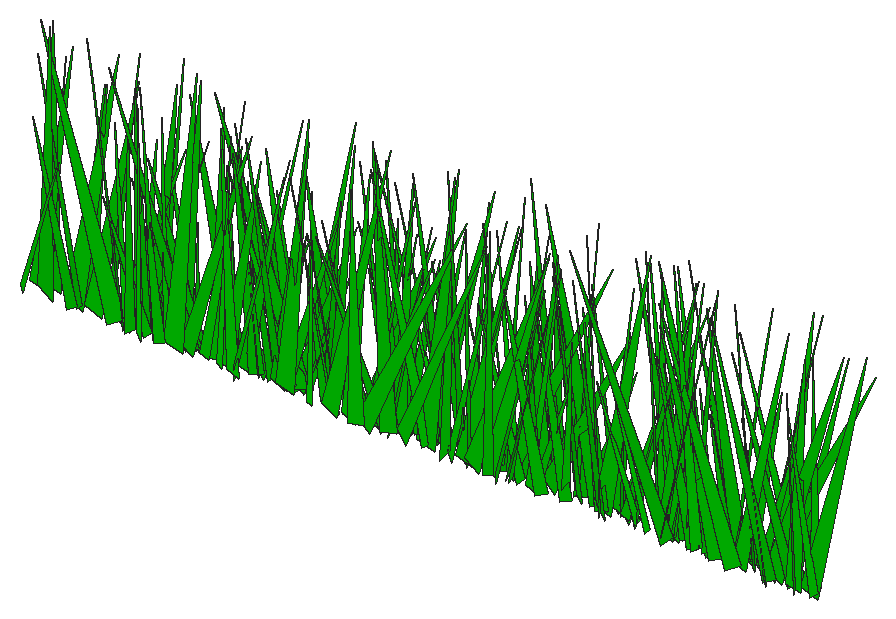
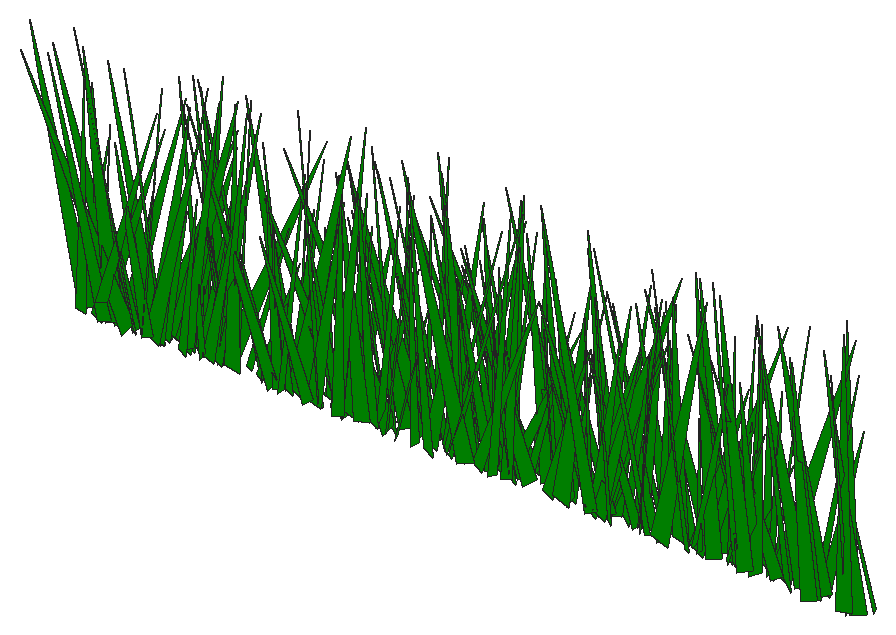
# SketchUp Ruby script. Lengths in inches.
U = 1.inch
M = Sketchup.active_model
def pt(a) = Geom::Point3d.new(a.map { |v| v * U })
def face(e, loops, mat)
  f = e.add_face(loops[0].map { |a| pt(a) })
  loops[1..].each { |l| e.add_face(l.map { |a| pt(a) }).erase! }
  f.material = f.back_material = mat if mat
  f
end
# faces: each face lists its corners as indices into pts; further lists are holes
def faces(e, pts, list, mat = nil) = list.each { |f| face(e, (f[0].is_a?(Array) ? f : [f]).map { |l| l.map { |i| pts[i] } }, mat) }
# xy, xz, yz: faces in a plane at the given z, y or x. An outline is a flat list of corners, or four numbers for a rectangle; further outlines are holes
def ring(l) = l.size == 4 ? [[l[0], l[1]], [l[2], l[1]], [l[2], l[3]], [l[0], l[3]]] : l.each_slice(2).to_a
def flat(e, list, mat, &to3) = list.each { |f| face(e, (f[0].is_a?(Array) ? f : [f]).map { |l| ring(l).map { |u, v| to3.(u, v) } }, mat) }
def xy(e, z, list, mat = nil) = flat(e, list, mat) { |x, y| [x, y, z] }
def xz(e, y, list, mat = nil) = flat(e, list, mat) { |x, z| [x, y, z] }
def yz(e, x, list, mat = nil) = flat(e, list, mat) { |y, z| [x, y, z] }
def lines(e, pts, list) = list.each { |a, b| e.add_line(pt(pts[a]), pt(pts[b])) }
# prism: a flat outline (further loops are holes) pulled along v
def prism(e, loops, v, mat = nil)
  f = face(e, loops, mat); d = Geom::Vector3d.new(v.map { |x| x * U })
  f.pushpull(f.normal.samedirection?(d) ? d.length : -d.length)
end
def box(e, o, s, mat = nil) = prism(e, [[o, [o[0] + s[0], o[1], o[2]], [o[0] + s[0], o[1] + s[1], o[2]], [o[0], o[1] + s[1], o[2]]]], [0, 0, s[2]], mat)
def at(x, y, z, deg = 0) = Geom::Transformation.translation(pt([x, y, z])) * Geom::Transformation.rotation(ORIGIN, Z_AXIS, deg.degrees)
def axes(o, x, y, z) = Geom::Transformation.new([*x, 0, *y, 0, *z, 0, *pt(o).to_a, 1])
def part(name) = M.definitions.add(name)
# library, detail: a bought-in or finely detailed component or shape, given as its bounding box
def library(name, o, s) = part(name).tap { |d| box(d.entities, o, s) }
def detail(e, o, s) = box(e.add_group.entities, o, s)
def put(e, d, t, mat = nil) = e.add_instance(d, t).tap { |i| i.material = mat if mat }
def group(e, t, mat = nil) = e.add_group.tap { |g| g.transformation = t; g.material = mat if mat }.entities
root = M.entities
M.materials.add("[Color G06]").color = [0, 204, 0]
c1 = part("fur_instance\#9")
p = [[0.8125,0,1.79],[0.67,-0.02,1.48],[0,-0.11,0],[0,0.11,0]]
faces(c1.entities,p,[[0,1,2,3]])
put(root,c1,axes([103.76,23.92,4.28],[-4.42176,-0.47384,0.10033],[-3.15087,0.57728,3.00292],[1.27403,-0.21685,7.7749]),"[Color G06]")
put(root,c1,axes([87.62,23.25,4.28],[0.67804,0.71547,0.05759],[5.07732,-0.09434,1.10789],[-0.7399,0.00827,7.65528]),"[Color G06]")
put(root,c1,axes([96.52,23.38,4.28],[3.3844,0.51064,1.9258],[3.53451,-0.50391,1.47424],[-1.60547,-0.03292,7.30528]),"[Color G06]")
put(root,c1,axes([100.07,23.5,4.28],[-1.47417,0.52641,1.3588],[3.79266,0.16613,1.79767],[-0.83244,-0.1753,5.78404]),"[Color G06]")
put(root,c1,axes([87.96,23.49,4.28],[4.85518,-0.52204,0.21187],[-3.35437,-0.59134,4.32478],[1.66845,0.33027,8.07829]),"[Color G06]")
put(root,c1,axes([101.4375,23.8,4.28],[2.62945,-0.37944,0.26273],[-2.61849,-0.36088,-1.33277],[-0.76066,-0.06937,5.49609]),"[Color G06]")
put(root,c1,axes([84.3125,23.48,4.28],[-2.87741,0.18491,1.60193],[1.12828,0.42631,-1.1257],[1.27832,0.03994,4.59942]),"[Color G06]")
put(root,c1,axes([64.55,23.6875,4.28],[3.14372,0.14643,0.49204],[1.09742,-0.40674,-1.75672],[0.08226,-0.16983,4.63175]),"[Color G06]")
put(root,c1,axes([96.36,23.67,4.28],[3.21126,-0.61959,0.94075],[-4.39498,-0.41239,2.31012],[0.90723,0.19533,7.8612]),"[Color G06]")
put(root,c1,axes([90.43,23.68,4.28],[4.64795,0.42794,0.1558],[2.83842,-0.58872,-3.39226],[1.17138,-0.27148,7.60175]),"[Color G06]")
put(root,c1,axes([95.21,23.64,4.28],[3.4759,-0.60332,0.87881],[-4.14978,-0.42387,3.23547],[1.35799,0.24898,7.63763]),"[Color G06]")
put(root,c1,axes([108.5,23.64,4.28],[-4.28972,-0.63093,0.37759],[-4.18755,0.53336,-3.88935],[-1.73207,0.27311,8.46797]),"[Color G06]")
put(root,c1,axes([97.49,23.87,4.28],[4.40916,-0.08799,0.02979],[-0.5859,-0.5776,-2.28566],[-0.2352,-0.21074,6.25226]),"[Color G06]")
put(root,c1,axes([86.02,23.81,4.28],[-3.0997,-0.11922,0.51967],[-0.72125,0.41891,1.42978],[0.57585,-0.11704,4.58809]),"[Color G06]")
put(root,c1,axes([115.39,23.71,4.28],[-2.96655,-0.61597,1.37495],[-4.43582,0.37004,-2.33493],[-0.82589,0.22506,7.60208]),"[Color G06]")
put(root,c1,axes([115.31,23.4375,4.28],[-3.58935,0.03386,0.73191],[-0.01334,0.44803,-2.52721],[0.54644,0.23335,4.74588]),"[Color G06]")
put(root,c1,axes([99.8,23.57,4.28],[-3.13994,-0.26934,2.44575],[-2.4014,0.43197,-1.42191],[0.80122,0.23914,5.32305]),"[Color G06]")
put(root,c1,axes([67.97,23.65,4.28],[-2.03674,-0.43572,1.74389],[-3.28522,0.2291,-1.99485],[-0.57664,0.23377,5.20544]),"[Color G06]")
put(root,c1,axes([97.06,23.38,4.28],[4.88819,0.10169,0.4948],[0.49771,-0.60941,3.40468],[-0.62748,0.30884,6.55518]),"[Color G06]")
put(root,c1,axes([85.55,23.61,4.28],[4.76013,-0.51297,2.32187],[-3.99265,-0.60567,2.91268],[0.06782,0.34741,8.50638]),"[Color G06]")
put(root,c1,axes([113.01,23.59,4.28],[-3.13676,0.64446,0.1265],[4.37802,0.40964,2.75959],[-1.48307,-0.15383,7.87875]),"[Color G06]")
put(root,c1,axes([72.71,23.47,4.28],[-4.5376,0.20348,2.07834],[0.91217,0.63323,-2.67342],[1.79751,0.19233,6.60317]),"[Color G06]")
put(root,c1,axes([99.12,23.64,4.28],[4.48387,-0.20567,1.93916],[-1.74673,-0.62372,1.42281],[-0.89868,0.18615,6.90973]),"[Color G06]")
put(root,c1,axes([94.34,23.92,4.28],[-5.00344,-0.43474,2.33291],[-2.92235,0.73056,1.63902],[1.9016,-0.02116,8.65712]),"[Color G06]")
put(root,c1,axes([65.85,24.06,4.28],[-3.13401,-0.74009,1.24941],[-5.02097,0.45146,2.58731],[1.91224,-0.02753,8.84115]),"[Color G06]")
put(root,c1,axes([101.53,23.74,4.28],[-1.94557,0.43929,1.45349],[3.28728,0.2464,1.27429],[-0.25275,-0.17687,5.38516]),"[Color G06]")
put(root,c1,axes([89.54,23.61,4.28],[1.67635,0.76745,2.44258],[5.5422,-0.27828,1.54748],[-1.49808,-0.17071,8.4582]),"[Color G06]")
put(root,c1,axes([99.52,23.74,4.28],[1.71601,0.29206,0.42477],[2.05227,-0.21803,-1.29917],[0.5055,-0.10628,3.83254]),"[Color G06]")
put(root,c1,axes([89.2,23.71,4.28],[-3.17243,-0.3846,0.3379],[-2.4927,0.37632,-3.07247],[-1.20191,0.23469,5.48027]),"[Color G06]")
put(root,c1,axes([79.1,23.47,4.28],[-3.88047,0.5135,0.37686],[3.53843,0.53204,-1.89308],[1.05057,0.10475,7.76809]),"[Color G06]")
put(root,c1,axes([106.99,23.83,4.28],[-3.27739,0.15455,0.50212],[1.15767,0.4411,1.28251],[0.03212,-0.12843,5.00922]),"[Color G06]")
put(root,c1,axes([92.07,23.81,4.28],[-4.76782,0.40055,1.23249],[2.9884,0.64053,1.9098],[0.02087,-0.21205,8.09697]),"[Color G06]")
put(root,c1,axes([110.25,23.94,4.28],[-4.93266,0.3144,3.52064],[2.88848,0.69769,1.88271],[1.5129,-0.307,7.88415]),"[Color G06]")
put(root,c1,axes([86.92,23.54,4.28],[-3.11873,0.60481,1.68165],[4.02012,0.46211,-2.43793],[1.97892,0.0144,7.60284]),"[Color G06]")
put(root,c1,axes([91.9375,23.82,4.28],[2.23973,0.72867,3.31468],[5.67106,-0.27248,-1.67866],[0.25161,-0.34488,8.32953]),"[Color G06]")
put(root,c1,axes([77.99,23.7,4.28],[4.45987,-0.08103,2.80629],[-1.00044,-0.65243,1.38749],[-1.69185,0.17221,6.57718]),"[Color G06]")
put(root,c1,axes([98.33,23.93,4.28],[-2.97416,0.28695,1.48091],[2.27672,0.35452,2.32259],[-0.18099,-0.25576,4.8809]),"[Color G06]")
put(root,c1,axes([117.11,23.66,4.28],[-3.9042,-0.02748,2.25127],[-0.71556,0.54423,-2.00895],[1.34005,0.21056,5.4863]),"[Color G06]")
put(root,c1,axes([87.95,23.87,4.28],[-3.50346,-0.29959,0.4492],[-2.16405,0.47706,-1.1511],[-0.15203,0.11332,6.03351]),"[Color G06]")
put(root,c1,axes([73.9375,23.68,4.28],[-0.02746,0.46538,0.10392],[3.2614,0.00167,1.06404],[-0.7115,-0.01029,4.87332]),"[Color G06]")
put(root,c1,axes([89.79,23.79,4.28],[-0.35765,0.44554,1.32908],[3.2079,0.01481,1.35783],[-0.84188,-0.13283,4.60927]),"[Color G06]")
put(root,c1,axes([118.22,23.98,4.28],[-3.19332,0.2203,1.89852],[1.9457,0.42584,1.63399],[0.56895,-0.21983,5.06788]),"[Color G06]")
put(root,c1,axes([117.85,24.04,4.28],[3.21385,-0.68495,0.78254],[-4.86617,-0.42401,2.0078],[0.84955,0.16245,8.54019]),"[Color G06]")
put(root,c1,axes([111.23,24.18,4.28],[1.26514,-0.68431,1.08413],[-4.3561,-0.20319,-3.37851],[-2.37333,0.00817,6.77897]),"[Color G06]")
put(root,c1,axes([109.63,24.04,4.28],[3.23534,-0.22781,1.37763],[-1.49286,-0.46788,-1.05646],[-1.13576,-0.03396,5.31294]),"[Color G06]")
put(root,c1,axes([71.97,23.6,4.28],[2.65898,0.50873,0.39153],[3.30744,-0.3537,2.62108],[-1.56181,0.11708,6.21722]),"[Color G06]")
put(root,c1,axes([78.24,23.88,4.28],[0.46601,0.60716,2.44774],[4.51254,-0.00324,-1.82685],[1.13024,-0.23742,6.28455]),"[Color G06]")
put(root,c1,axes([81.71,24.15,4.28],[-4.21965,-0.44122,0.67658],[-3.07984,0.58922,1.23426],[0.85497,-0.05507,7.78541]),"[Color G06]")
put(root,c1,axes([73.33,24.17,4.28],[-4.90448,0.08045,3.27223],[1.34534,0.68942,2.55703],[1.82111,-0.29264,6.92354]),"[Color G06]")
put(root,c1,axes([89.38,24.25,4.28],[1.1707,-0.82951,0.612],[-5.88988,-0.16994,-1.29294],[-0.929,0.03211,8.96846]),"[Color G06]")
put(root,c1,axes([113.16,23.97,4.28],[4.07167,-0.49988,1.52813],[-3.72743,-0.54327,1.76992],[0.04742,0.21807,7.9123]),"[Color G06]")
put(root,c1,axes([94.97,23.6875,4.28],[4.14644,0.35157,2.25261],[1.9006,-0.59833,2.91269],[-2.23961,0.14314,6.64228]),"[Color G06]")
put(root,c1,axes([87.83,24.11,4.28],[5.1232,0.20366,1.42002],[1.69092,-0.6804,-2.41716],[-0.42021,-0.25491,7.58629]),"[Color G06]")
put(root,c1,axes([94.58,23.74,4.28],[2.45833,0.71801,0.27765],[5.09389,-0.33438,-1.41188],[0.77401,-0.07984,8.40999]),"[Color G06]")
put(root,c1,axes([93.68,23.68,4.28],[5.80096,-0.01851,1.26512],[-0.45997,-0.74883,3.45243],[-0.7229,0.32792,7.95539]),"[Color G06]")
put(root,c1,axes([108.4,24.14,4.28],[5.37383,-0.30532,1.30049],[-2.09826,-0.75762,-1.06512],[-1.07163,-0.04762,8.607]),"[Color G06]")
put(root,c1,axes([85.29,24.11,4.28],[-4.68156,-0.04223,0.93887],[-0.16996,0.6457,1.44358],[0.67636,-0.13007,6.86134]),"[Color G06]")
put(root,c1,axes([89.65,23.63,4.28],[4.83158,0.28922,0.16745],[1.85445,-0.61846,3.18786],[-0.93568,0.26774,7.18276]),"[Color G06]")
put(root,c1,axes([88.24,23.99,4.28],[3.31274,-0.40924,0.39635],[-2.82575,-0.4254,2.29897],[0.83572,0.18383,6.20224]),"[Color G06]")
put(root,c1,axes([72.9375,23.91,4.28],[-1.24194,0.38027,0.07727],[2.44966,0.15203,2.00087],[-1.19937,-0.08325,4.00668]),"[Color G06]")
put(root,c1,axes([79.1,23.5625,4.28],[5.74462,0.11844,0.75404],[0.44151,-0.67914,4.74091],[-0.88377,0.4306,7.26984]),"[Color G06]")
put(root,c1,axes([80.09,24.22,4.28],[0.95988,-0.65182,0.91207],[-4.57913,-0.14955,-1.51282],[-1.11956,0.05284,6.96963]),"[Color G06]")
put(root,c1,axes([94.25,24.21,4.28],[5.80567,-0.15792,0.06654],[-1.1003,-0.79313,-1.78664],[-0.27167,-0.16245,8.65812]),"[Color G06]")
put(root,c1,axes([75.82,24.12,4.28],[-3.95512,-0.62765,0.07684],[-4.31073,0.52539,-2.64285],[-1.29596,0.16792,8.55639]),"[Color G06]")
put(root,c1,axes([75.58,23.93,4.28],[3.478,0.57392,0.58913],[4.0545,-0.45937,-2.06023],[0.80974,-0.16499,7.78551]),"[Color G06]")
put(root,c1,axes([110.01,23.95,4.28],[-0.95496,0.51654,1.25604],[3.66451,0.09348,1.80706],[-0.99968,-0.15076,5.42424]),"[Color G06]")
put(root,c1,axes([103.78,23.77,4.28],[-5.53145,-0.03072,3.00833],[-0.94951,0.76053,-3.00777],[1.78842,0.30877,7.70763]),"[Color G06]")
put(root,c1,axes([97.8,23.74,4.28],[5.24647,0.3102,0.91221],[1.95299,-0.70985,2.63934],[-1.22757,0.19642,8.0977]),"[Color G06]")
put(root,c1,axes([81.65,24.09,4.28],[-1.68321,-0.63032,3.60073],[-4.72987,0.32699,1.63664],[1.96588,0.24705,7.02071]),"[Color G06]")
put(root,c1,axes([85.28,24.21,4.28],[4.35517,0.42056,3.49805],[3.68826,-0.59132,-2.09053],[-0.98529,-0.35452,7.63655]),"[Color G06]")
put(root,c1,axes([73.95,24.23,4.28],[-4.20785,0.08472,3.23099],[1.23213,0.6224,1.70972],[1.87733,-0.21861,6.11981]),"[Color G06]")
put(root,c1,axes([68.25,23.98,4.28],[-4.75983,-0.23493,1.48367],[-1.89001,0.64617,-1.79059],[0.50169,0.20537,7.33088]),"[Color G06]")
put(root,c1,axes([82.25,23.94,4.28],[0.14072,0.78556,2.23618],[5.78272,0.00736,-1.10992],[0.73109,-0.20943,8.34876]),"[Color G06]")
put(root,c1,axes([70.74,23.96,4.28],[-2.81685,0.77509,1.03789],[5.34422,0.33938,3.28429],[-1.67853,-0.2202,8.71499]),"[Color G06]")
put(root,c1,axes([105.72,24.26,4.28],[6.03573,0.19538,0.91676],[1.52571,-0.79357,-3.00977],[-0.10748,-0.29317,8.75796]),"[Color G06]")
put(root,c1,axes([76.7,24.04,4.28],[4.14069,-0.3042,1.59392],[-2.38059,-0.56649,1.39463],[-0.47851,0.186,6.85445]),"[Color G06]")
put(root,c1,axes([93.43,23.59,4.28],[4.51513,0.60583,0.41259],[3.7387,-0.56804,4.42505],[-2.23019,0.27427,8.25348]),"[Color G06]")
put(root,c1,axes([74.82,23.76,4.28],[-1.38709,0.84486,0.43069],[5.94579,0.19754,-1.74016],[1.19934,-0.0022,9.12501]),"[Color G06]")
put(root,c1,axes([115.25,24.26,4.28],[2.7128,-0.72957,0.38909],[-4.98924,-0.34739,2.87559],[1.59646,0.15408,8.32558]),"[Color G06]")
put(root,c1,axes([116.68,24.08,4.28],[-3.2046,-0.4911,1.19305],[-3.50191,0.3863,-2.74461],[-0.88153,0.25071,6.56599]),"[Color G06]")
put(root,c1,axes([116.86,23.92,4.28],[-1.96966,0.61703,1.4597],[4.38052,0.29727,-1.23192],[1.15956,-0.07492,7.13333]),"[Color G06]")
put(root,c1,axes([72.83,24.04,4.28],[-3.97739,-0.29762,2.82201],[-2.5434,0.57464,-1.04552],[1.28512,0.21616,6.66477]),"[Color G06]")
put(root,c1,axes([79.35,24.1875,4.28],[3.00418,-0.47702,0.93058],[-3.47321,-0.40631,1.12042],[0.16327,0.13397,6.71149]),"[Color G06]")
put(root,c1,axes([111.8,23.89,4.28],[-1.29344,0.84878,0.79293],[5.80688,0.14725,3.05159],[-1.90026,-0.12775,8.78543]),"[Color G06]")
put(root,c1,axes([71.31,23.87,4.28],[-5.90892,-0.02345,1.82867],[-0.59143,0.78582,-3.11133],[1.08422,0.30087,8.26891]),"[Color G06]")
put(root,c1,axes([107.98,24.17,4.28],[-1.6969,-0.66107,3.66484],[-4.96681,0.32694,1.63749],[1.95391,0.25695,7.34524]),"[Color G06]")
put(root,c1,axes([101.95,24.34,4.28],[-4.53463,-0.29903,1.2541],[-1.9433,0.63558,1.71338],[1.23538,-0.09783,7.29853]),"[Color G06]")
put(root,c1,axes([91.7,24.14,4.28],[4.00061,0.37651,1.4035],[2.84316,-0.54751,-1.22995],[-0.29796,-0.16909,7.10797]),"[Color G06]")
put(root,c1,axes([103.66,24.17,4.28],[3.38788,-0.65218,2.06153],[-4.86451,-0.43592,2.01534],[0.33594,0.26487,8.39269]),"[Color G06]")
put(root,c1,axes([105.99,24.22,4.28],[-2.78166,0.15925,0.37421],[1.15011,0.35652,1.66772],[-0.21018,-0.15675,4.17325]),"[Color G06]")
put(root,c1,axes([72.01,24.55,4.28],[-3.33455,-0.67078,0.05543],[-4.52992,0.43997,2.90772],[1.61888,-0.15055,8.2505]),"[Color G06]")
put(root,c1,axes([94.26,24.36,4.28],[-0.13404,-0.5905,0.32918],[-4.10367,0.01033,-1.60494],[-1.06801,0.03444,6.1254]),"[Color G06]")
put(root,c1,axes([93.22,24.11,4.28],[2.69734,0.56692,4.08087],[4.14738,-0.4956,1.78571],[-2.60448,-0.20206,7.06994]),"[Color G06]")
put(root,c1,axes([112.48,24.1,4.28],[0.44033,0.38785,1.46671],[2.7488,-0.10412,1.31954],[-1.06918,-0.10796,3.99652]),"[Color G06]")
put(root,c1,axes([107.65,23.99,4.28],[-5.5403,0.05647,2.73888],[-0.01512,0.79511,-1.95164],[1.8767,0.17312,8.06984]),"[Color G06]")
put(root,c1,axes([110.02,24.1875,4.28],[-2.80623,-0.32436,1.03163],[-2.42548,0.37883,-1.05515],[0.06282,0.1374,5.34443]),"[Color G06]")
put(root,c1,axes([110.86,24.04,4.28],[1.67743,0.4586,1.57953],[3.091,-0.27241,1.75306],[-1.54216,-0.04718,5.23177]),"[Color G06]")
put(root,c1,axes([71.51,23.89,4.28],[-4.04072,0.31011,0.4785],[1.94439,0.52868,-2.68227],[1.12578,0.19995,6.35012]),"[Color G06]")
put(root,c1,axes([76.14,24.43,4.28],[-0.24287,-0.60224,0.05194],[-3.97966,0.02932,-2.51445],[-1.67799,0.01763,5.95597]),"[Color G06]")
put(root,c1,axes([82.48,24.21,4.28],[-3.70641,0.36206,0.20705],[2.50946,0.48932,2.05325],[-0.68047,-0.16754,6.44427]),"[Color G06]")
put(root,c1,axes([89.98,23.95,4.28],[2.53746,0.67643,0.76922],[4.8021,-0.3606,1.04271],[-0.85753,-0.01778,8.11522]),"[Color G06]")
put(root,c1,axes([107.79,24.01,4.28],[5.57284,0.13794,0.65542],[0.872,-0.76247,1.87212],[-0.64065,0.16208,8.24945]),"[Color G06]")
put(root,c1,axes([87.6,24.25,4.28],[0.47795,-0.63035,2.81125],[-4.26138,0.07622,3.58146],[2.41093,0.25967,5.77301]),"[Color G06]")
put(root,c1,axes([109.71,24.4375,4.28],[5.26442,0.2026,3.00847],[2.10047,-0.71429,-2.68441],[-1.32319,-0.32783,7.70816]),"[Color G06]")
put(root,c1,axes([86.18,24.02,4.28],[3.35523,0.15927,1.48894],[0.67364,-0.45902,2.24947],[-1.35764,0.16585,4.79587]),"[Color G06]")
put(root,c1,axes([84.6,24.56,4.28],[-3.53955,-0.4625,1.77798],[-2.55504,0.4988,3.54342],[2.42647,-0.14944,6.32475]),"[Color G06]")
put(root,c1,axes([108.4,24.06,4.28],[2.85302,0.22323,0.31304],[1.4961,-0.38784,1.31363],[-0.60692,0.09334,4.70968]),"[Color G06]")
put(root,c1,axes([99.51,24.53,4.28],[1.83226,-0.64786,0.63338],[-4.51586,-0.26223,-1.63219],[-1.17129,-0.00243,7.28364]),"[Color G06]")
put(root,c1,axes([107.62,24.47,4.28],[3.40961,-0.59768,1.76257],[-4.19822,-0.50108,-1.37797],[-1.46176,0.04499,8.06882]),"[Color G06]")
put(root,c1,axes([70.86,24.14,4.28],[2.22558,0.57585,0.10584],[3.884,-0.28799,-2.43788],[1.40456,-0.11607,6.5737]),"[Color G06]")
put(root,c1,axes([105.06,24.36,4.28],[1.13649,-0.34888,0.14792],[-2.38613,-0.14632,1.30843],[0.75879,0.06243,3.89301]),"[Color G06]")
put(root,c1,axes([103.67,24.1,4.28],[-0.25908,0.58691,0.69136],[4.16504,0.02369,1.17641],[-0.76243,-0.07004,6.19165]),"[Color G06]")
put(root,c1,axes([82.12,24.18,4.28],[2.44072,0.50646,0.29773],[3.53476,-0.32235,-1.73642],[0.85818,-0.11269,6.30536]),"[Color G06]")
put(root,c1,axes([108.93,24.33,4.28],[2.24868,0.56717,4.90446],[4.45908,-0.46803,1.65075],[-2.72551,-0.29777,6.74715]),"[Color G06]")
put(root,c1,axes([89.91,24.27,4.28],[-1.46855,0.37647,2.59508],[2.81091,0.27939,-1.10285],[1.54993,-0.15,4.45894]),"[Color G06]")
put(root,c1,axes([80.26,24.17,4.28],[-4.25896,0.0037,1.67876],[-0.22869,0.59833,-1.44754],[1.10003,0.13872,6.19867]),"[Color G06]")
put(root,c1,axes([72.65,24.21,4.28],[4.88637,-0.04573,0.00223],[-0.32317,-0.67087,1.2806],[0.05591,0.11923,7.20658]),"[Color G06]")
put(root,c1,axes([89.29,24.38,4.28],[-5.24248,0.04478,1.83981],[0.49837,0.74201,1.09733],[1.17051,-0.11535,7.77289]),"[Color G06]")
put(root,c1,axes([75.875,24.48,4.28],[-2.24038,-0.26321,0.86732],[-1.57877,0.31225,1.77614],[1.18622,-0.08154,4.00198]),"[Color G06]")
put(root,c1,axes([74.85,24.51,4.28],[-1.91116,-0.75759,2.04927],[-5.3213,0.30867,2.02337],[1.75504,0.11091,8.36642]),"[Color G06]")
put(root,c1,axes([69.14,24.09,4.28],[0.579,0.75453,0.83722],[5.29026,-0.0598,-1.98086],[1.267,-0.0951,7.88832]),"[Color G06]")
put(root,c1,axes([114.26,24.38,4.28],[2.59253,0.30827,1.20995],[2.32375,-0.30812,-2.10387],[0.37782,-0.22023,4.63724]),"[Color G06]")
put(root,c1,axes([82.96,24.39,4.28],[-1.38086,0.76135,3.96462],[5.49209,-0.00487,4.38025],[-2.58531,-0.41699,7.18758]),"[Color G06]")
put(root,c1,axes([91.64,24.43,4.28],[1.0598,-0.77126,2.26061],[-5.70279,-0.11944,1.29104],[0.59717,0.22817,8.31709]),"[Color G06]")
put(root,c1,axes([80.19,24.41,4.28],[2.60531,0.35339,1.14941],[2.53595,-0.28952,-2.61435],[0.76346,-0.24426,4.76163]),"[Color G06]")
put(root,c1,axes([81.96,24.5,4.28],[3.41419,-0.08749,0.82931],[-0.44869,-0.46527,-1.51243],[-0.70726,-0.12717,4.96286]),"[Color G06]")
put(root,c1,axes([97.05,24.6,4.28],[-5.02139,-0.21694,1.58454],[-1.20028,0.69334,2.40803],[1.45038,-0.17728,7.47865]),"[Color G06]")
put(root,c1,axes([91.88,24.33,4.28],[2.77879,-0.37485,1.18531],[-2.78928,-0.35463,1.72315],[0.27425,0.19135,5.51551]),"[Color G06]")
put(root,c1,axes([103.68,24.56,4.28],[4.87694,-0.23802,1.00121],[-1.53442,-0.67507,-1.74024],[-1.00389,-0.12447,7.52385]),"[Color G06]")
put(root,c1,axes([72.67,24.62,4.28],[-1.68628,-0.76405,1.51596],[-5.21632,0.26842,2.57965],[1.95979,0.05702,8.17059]),"[Color G06]")
put(root,c1,axes([112.87,24.48,4.28],[-0.20959,-0.70204,1.9888],[-5.08615,-0.01224,-1.6936],[-1.11707,0.18745,7.33803]),"[Color G06]")
put(root,c1,axes([90.09,24.22,4.28],[-3.08228,0.10643,1.63971],[0.41569,0.44184,-1.54903],[1.27019,0.11367,4.48591]),"[Color G06]")
put(root,c1,axes([89.3,24.1875,4.28],[2.52607,0.50631,1.15314],[3.55794,-0.36736,1.11909],[-1.0582,-0.02651,6.51534]),"[Color G06]")
put(root,c1,axes([84.72,24.3,4.28],[-0.12173,0.39354,1.06739],[2.8061,-0.01067,1.16687],[-0.77498,-0.10046,4.05743]),"[Color G06]")
put(root,c1,axes([81.08,24.23,4.28],[-4.56452,-0.29537,2.19069],[-2.51467,0.6011,-2.39369],[0.55824,0.29257,7.12968]),"[Color G06]")
put(root,c1,axes([113.93,24.22,4.28],[-5.20587,0.01683,2.28709],[-0.21277,0.7393,-1.70684],[1.5202,0.16111,7.59318]),"[Color G06]")
put(root,c1,axes([78.3125,24.59,4.28],[1.77061,-0.3364,0.00566],[-2.29751,-0.23534,-1.35994],[-0.73568,-0.07467,4.26068]),"[Color G06]")
put(root,c1,axes([96.88,24.25,4.28],[5.28378,0.28872,2.31783],[1.94356,-0.76763,1.0874],[-1.7072,0.01968,8.41165]),"[Color G06]")
put(root,c1,axes([93.25,24.34,4.28],[-5.27753,-0.16651,0.64258],[-1.25211,0.72497,-1.39083],[0.20709,0.14,7.96653]),"[Color G06]")
put(root,c1,axes([104.87,24.54,4.28],[4.77572,0.49743,1.11177],[3.43362,-0.55705,-4.31574],[1.22007,-0.37941,7.79392]),"[Color G06]")
put(root,c1,axes([97.07,24.32,4.28],[4.79289,-0.54612,0.26122],[-3.49017,-0.5769,4.49452],[1.78527,0.33833,8.0854]),"[Color G06]")
put(root,c1,axes([74.07,24.36,4.28],[-3.17448,-0.11322,0.23901],[-0.82688,0.43055,-1.10362],[-0.03224,0.10526,4.77124]),"[Color G06]")
put(root,c1,axes([82.69,24.47,4.28],[2.33123,-0.51415,0.6025],[-3.48876,-0.28142,2.56592],[1.25924,0.17216,5.99355]),"[Color G06]")
put(root,c1,axes([83.52,24.34,4.28],[3.1756,-0.08624,0.01822],[-0.5964,-0.4245,1.37321],[0.16417,0.12607,4.63625]),"[Color G06]")
put(root,c1,axes([67.75,24.15,4.28],[-1.38649,0.78643,1.37925],[5.32474,0.22586,-2.83744],[2.07494,-0.0541,8.2031]),"[Color G06]")
put(root,c1,axes([88.42,24.64,4.28],[4.36526,-0.23296,0.20805],[-1.59442,-0.59367,-1.63613],[-0.51784,-0.13589,6.79137]),"[Color G06]")
put(root,c1,axes([76.13,24.4,4.28],[-2.66554,0.37875,1.08816],[2.81202,0.35849,1.05252],[-0.01059,-0.14124,5.58952]),"[Color G06]")
put(root,c1,axes([108.48,24.2,4.28],[-5.16678,0.37264,1.09738],[2.48992,0.7193,-1.87161],[1.21674,0.1104,8.48997]),"[Color G06]")
put(root,c1,axes([117.87,24.57,4.28],[3.74107,-0.37673,2.34111],[-2.61505,-0.56423,-1.09559],[-1.70699,0.03874,6.80924]),"[Color G06]")
put(root,c1,axes([99.76,24.48,4.28],[2.59035,-0.55824,0.42092],[-3.4618,-0.28717,3.83693],[2.03021,0.2226,6.00545]),"[Color G06]")
put(root,c1,axes([88.82,24.7,4.28],[-3.22812,-0.54475,0.98114],[-3.78111,0.45894,1.48288],[1.1813,-0.01967,7.42754]),"[Color G06]")
put(root,c1,axes([85.08,24.77,4.28],[1.20094,-0.69998,0.22186],[-4.81923,-0.16662,-2.11853],[-1.41236,-0.02665,7.41747]),"[Color G06]")
put(root,c1,axes([77.41,24.15,4.28],[1.8711,0.73779,0.25526],[5.22971,-0.26154,1.21065],[-0.82038,0.01546,8.29974]),"[Color G06]")
put(root,c1,axes([109.28,24.46,4.28],[-0.64188,-0.41869,1.99706],[-3.19851,0.03596,-1.43024],[-0.75516,0.20356,4.36034]),"[Color G06]")
put(root,c1,axes([113.04,24.59,4.28],[-1.45611,-0.63623,1.18033],[-4.50671,0.16822,-2.00258],[-1.06319,0.1583,6.87212]),"[Color G06]")
put(root,c1,axes([101.55,24.62,4.28],[5.68597,-0.15459,2.28079],[-0.94383,-0.81834,-1.11573],[-1.63309,-0.06528,8.58592]),"[Color G06]")
put(root,c1,axes([103.21,24.45,4.28],[-0.30341,-0.74822,4.31308],[-5.78645,-0.09071,-2.71692],[-1.90674,0.39434,7.55878]),"[Color G06]")
put(root,c1,axes([114.16,24.62,4.28],[6.21125,0.03539,0.68397],[0.32411,-0.85696,-1.48061],[-0.41086,-0.14097,9.17218]),"[Color G06]")
put(root,c1,axes([92.7,24.63,4.28],[-6.11596,0.00801,0.18506],[0.07684,0.84166,1.485],[0.11283,-0.13873,9.01972]),"[Color G06]")
put(root,c1,axes([72.22,24.26,4.28],[-1.51163,0.56845,0.29749],[3.94501,0.21109,-1.55883],[1.04613,0.02536,6.30828]),"[Color G06]")
put(root,c1,axes([104.84,24.38,4.28],[3.02767,0.17863,1.75593],[0.99933,-0.44812,1.38786],[-1.42219,0.0654,4.71336]),"[Color G06]")
put(root,c1,axes([104.41,24.61,4.28],[-1.56448,-0.47238,1.89664],[-3.40137,0.25773,1.10655],[1.23146,0.11174,5.4659]),"[Color G06]")
put(root,c1,axes([78.18,24.8,4.28],[-2.99438,-0.47283,0.61069],[-3.15503,0.41198,2.0859],[1.30766,-0.08872,6.43114]),"[Color G06]")
put(root,c1,axes([98.7,24.64,4.28],[1.02071,-0.66769,1.64388],[-4.88613,-0.12165,1.10111],[0.51181,0.17025,7.23372]),"[Color G06]")
put(root,c1,axes([114.65,24.59,4.28],[4.30111,0.62233,0.51364],[3.90217,-0.48876,-4.96217],[2.19291,-0.35091,7.82249]),"[Color G06]")
put(root,c1,axes([65.83,24.72,4.28],[-2.22261,-0.73075,1.85559],[-5.24794,0.33594,1.15639],[1.20933,0.11479,8.42855]),"[Color G06]")
put(root,c1,axes([65.07,24.47,4.28],[-0.27247,0.69648,2.85566],[5.16293,0.10377,-1.80691],[1.39325,-0.24832,7.25428]),"[Color G06]")
put(root,c1,axes([86.08,24.64,4.28],[-1.38281,-0.46241,0.5709],[-3.21868,0.16943,-1.64961],[-0.88454,0.10636,5.11011]),"[Color G06]")
put(root,c1,axes([104.08,24.8125,4.28],[-4.21332,-0.36521,0.87336],[-2.38452,0.57913,2.12352],[1.23077,-0.12821,7.10395]),"[Color G06]")
put(root,c1,axes([100.29,24.53,4.28],[1.34174,0.44683,1.48181],[3.30261,-0.14997,-1.48482],[0.58603,-0.17784,4.97514]),"[Color G06]")
put(root,c1,axes([97.71,24.35,4.28],[-4.63969,0.27239,1.20043],[1.76392,0.64842,-1.67346],[1.16169,0.10335,7.33542]),"[Color G06]")
put(root,c1,axes([82.87,24.33,4.28],[-1.5666,0.6708,0.25359],[4.75874,0.2121,1.21843],[-0.72375,-0.05742,7.46243]),"[Color G06]")
put(root,c1,axes([110.88,24.27,4.28],[-4.99429,0.47167,0.3424],[3.29433,0.68861,-1.63585],[0.80075,0.10885,8.86552]),"[Color G06]")
put(root,c1,axes([89.67,24.84,4.28],[-4.39266,-0.51899,1.29354],[-3.50033,0.62028,2.037],[1.53252,-0.07083,8.36023]),"[Color G06]")
put(root,c1,axes([91.59,24.74,4.28],[3.81314,-0.69495,0.29072],[-4.91499,-0.5178,1.81179],[0.84725,0.12391,9.20196]),"[Color G06]")
put(root,c1,axes([112.41,24.38,4.28],[5.39636,0.2395,1.29928],[1.55361,-0.7549,1.57161],[-1.13663,0.10524,8.31671]),"[Color G06]")
put(root,c1,axes([90.05,24.48,4.28],[1.46374,0.50485,0.97675],[3.6356,-0.18349,-1.27539],[0.5631,-0.12767,5.69547]),"[Color G06]")
put(root,c1,axes([101.93,24.68,4.28],[-1.36562,-0.58579,1.44092],[-4.28918,0.17083,-1.10233],[-0.42407,0.1586,6.50926]),"[Color G06]")
put(root,c1,axes([92.11,24.29,4.28],[3.38951,0.26537,1.19349],[1.31111,-0.44224,2.97824],[-1.59377,0.20055,4.98824]),"[Color G06]")
put(root,c1,axes([116.19,24.67,4.28],[4.3325,-0.46963,0.50457],[-3.37499,-0.5936,1.26437],[0.25683,0.12186,8.10349]),"[Color G06]")
put(root,c1,axes([94.96,24.84,4.28],[-3.04744,-0.45286,1.31023],[-2.8493,0.43519,2.47567],[1.78793,-0.07834,6.17852]),"[Color G06]")
put(root,c1,axes([90.85,24.65,4.28],[-3.1989,-0.43159,0.10478],[-2.97813,0.42516,-1.921],[-0.84561,0.13533,6.36912]),"[Color G06]")
put(root,c1,axes([83.125,24.69,4.28],[-1.47526,-0.52535,0.98225],[-3.64991,0.16409,-2.16347],[-1.14179,0.15425,5.64675]),"[Color G06]")
put(root,c1,axes([116.73,24.65,4.28],[-4.40482,0.36174,0.7869],[2.63598,0.58646,1.99015],[-0.24129,-0.19682,7.3764]),"[Color G06]")
put(root,c1,axes([112.48,24.39,4.28],[-6.14753,0.02977,1.25187],[-0.0353,0.82952,-2.6531],[0.86367,0.24579,8.80232]),"[Color G06]")
put(root,c1,axes([78.27,24.87,4.28],[-0.99619,-0.77685,0.63581],[-5.47002,0.12333,-1.83416],[-1.13836,0.08721,8.25707]),"[Color G06]")
put(root,c1,axes([113.3125,24.62,4.28],[-0.58408,-0.46785,2.96106],[-3.59753,0.17205,1.53758],[1.49649,0.231,4.85202]),"[Color G06]")
put(root,c1,axes([110.83,24.77,4.28],[-2.66392,0.19589,2.32051],[1.94716,0.36058,1.49648],[0.76979,-0.23419,4.24503]),"[Color G06]")
put(root,c1,axes([67.89,24.73,4.28],[-0.57791,-0.63194,2.25687],[-4.62964,0.12634,1.4158],[1.17655,0.18674,6.67962]),"[Color G06]")
put(root,c1,axes([82.49,24.72,4.28],[-0.30077,-0.52383,1.69878],[-3.67412,-0.01831,-2.10158],[-1.37985,0.16293,5.22555]),"[Color G06]")
put(root,c1,axes([76.48,24.78,4.28],[5.55738,-0.13009,1.45951],[-0.80354,-0.78198,-1.17224],[-1.08547,-0.08715,8.34015]),"[Color G06]")
put(root,c1,axes([83.05,24.72,4.28],[4.49263,0.55161,2.45821],[4.28322,-0.58491,-2.40829],[-0.08456,-0.32086,8.6162]),"[Color G06]")
put(root,c1,axes([73.38,24.47,4.28],[-4.68661,-0.2025,5.16202],[-2.43187,0.75116,-1.54681],[2.85025,0.30793,7.16804]),"[Color G06]")
put(root,c1,axes([68.07,24.95,4.28],[-0.535,-0.72874,0.30953],[-5.08847,0.07924,1.7838],[1.20877,0.01102,7.6461]),"[Color G06]")
put(root,c1,axes([69.95,24.38,4.28],[5.09713,0.42191,1.09461],[2.77065,-0.70418,2.3605],[-1.41934,0.14058,8.53883]),"[Color G06]")
put(root,c1,axes([100.38,24.65,4.28],[-4.6153,-0.5164,3.00919],[-4.10397,0.6455,-1.33524],[0.9618,0.27633,8.7425]),"[Color G06]")
put(root,c1,axes([81.65,24.89,4.28],[4.50695,-0.10582,1.69359],[-0.39882,-0.62399,-2.10821],[-1.30418,-0.17488,6.49732]),"[Color G06]")
put(root,c1,axes([98.17,24.4375,4.28],[3.16648,0.55832,0.78175],[3.8753,-0.44624,1.54765],[-1.13418,0.03402,7.47062]),"[Color G06]")
put(root,c1,axes([83.3,24.4375,4.28],[3.82581,0.28538,1.61803],[1.53049,-0.53052,2.66542],[-1.73723,0.16109,5.91154]),"[Color G06]")
put(root,c1,axes([100.125,24.92,4.28],[-2.23413,-0.5734,0.94109],[-4.01687,0.32327,1.3258],[1.08164,0.01617,6.86743]),"[Color G06]")
put(root,c1,axes([115.67,24.4,4.28],[-1.1951,0.8322,0.75078],[5.80347,0.17856,-2.10145],[1.47933,-0.0282,8.85056]),"[Color G06]")
put(root,c1,axes([79.77,24.61,4.28],[-3.66436,0.03042,1.81856],[-0.03198,0.5283,-1.15907],[1.23576,0.10387,5.36251]),"[Color G06]")
put(root,c1,axes([102.28,24.77,4.28],[1.52976,-0.43199,0.60705],[-2.89471,-0.17222,2.21568],[1.17597,0.13803,4.66433]),"[Color G06]")
put(root,c1,axes([96.14,24.9375,4.28],[-3.52653,-0.16011,0.03863],[-1.08285,0.46741,1.73497],[0.38274,-0.15287,5.26447]),"[Color G06]")
put(root,c1,axes([65.76,24.53,4.28],[4.77611,0.01918,2.67153],[-0.44143,-0.67487,2.31939],[-1.73758,0.22417,6.75406]),"[Color G06]")
put(root,c1,axes([79.22,24.74,4.28],[5.42681,0.27141,1.07464],[2.02969,-0.75267,-1.05857],[-0.43073,-0.12728,8.55136]),"[Color G06]")
put(root,c1,axes([82.8125,24.66,4.28],[-0.25274,0.53794,1.48314],[3.8828,0.00232,1.38112],[-0.88901,-0.14278,5.61046]),"[Color G06]")
put(root,c1,axes([93.83,25.05,4.28],[5.27737,-0.34476,1.07609],[-2.2027,-0.72297,-2.47824],[-1.33385,-0.17014,8.35008]),"[Color G06]")
